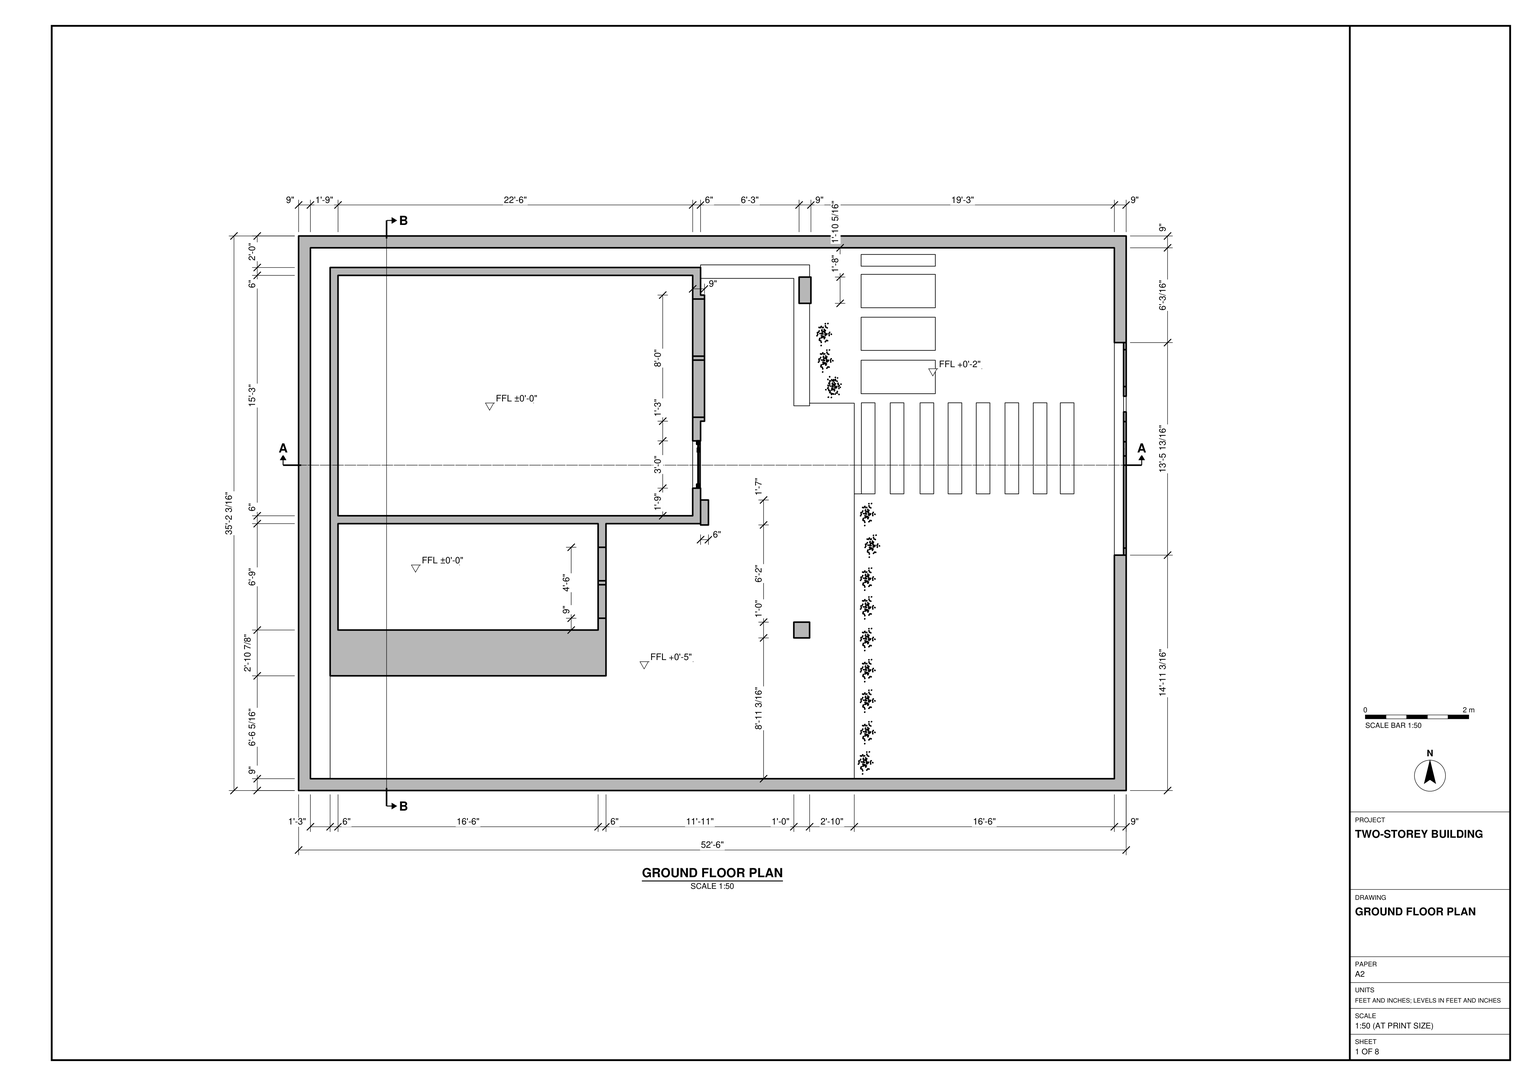
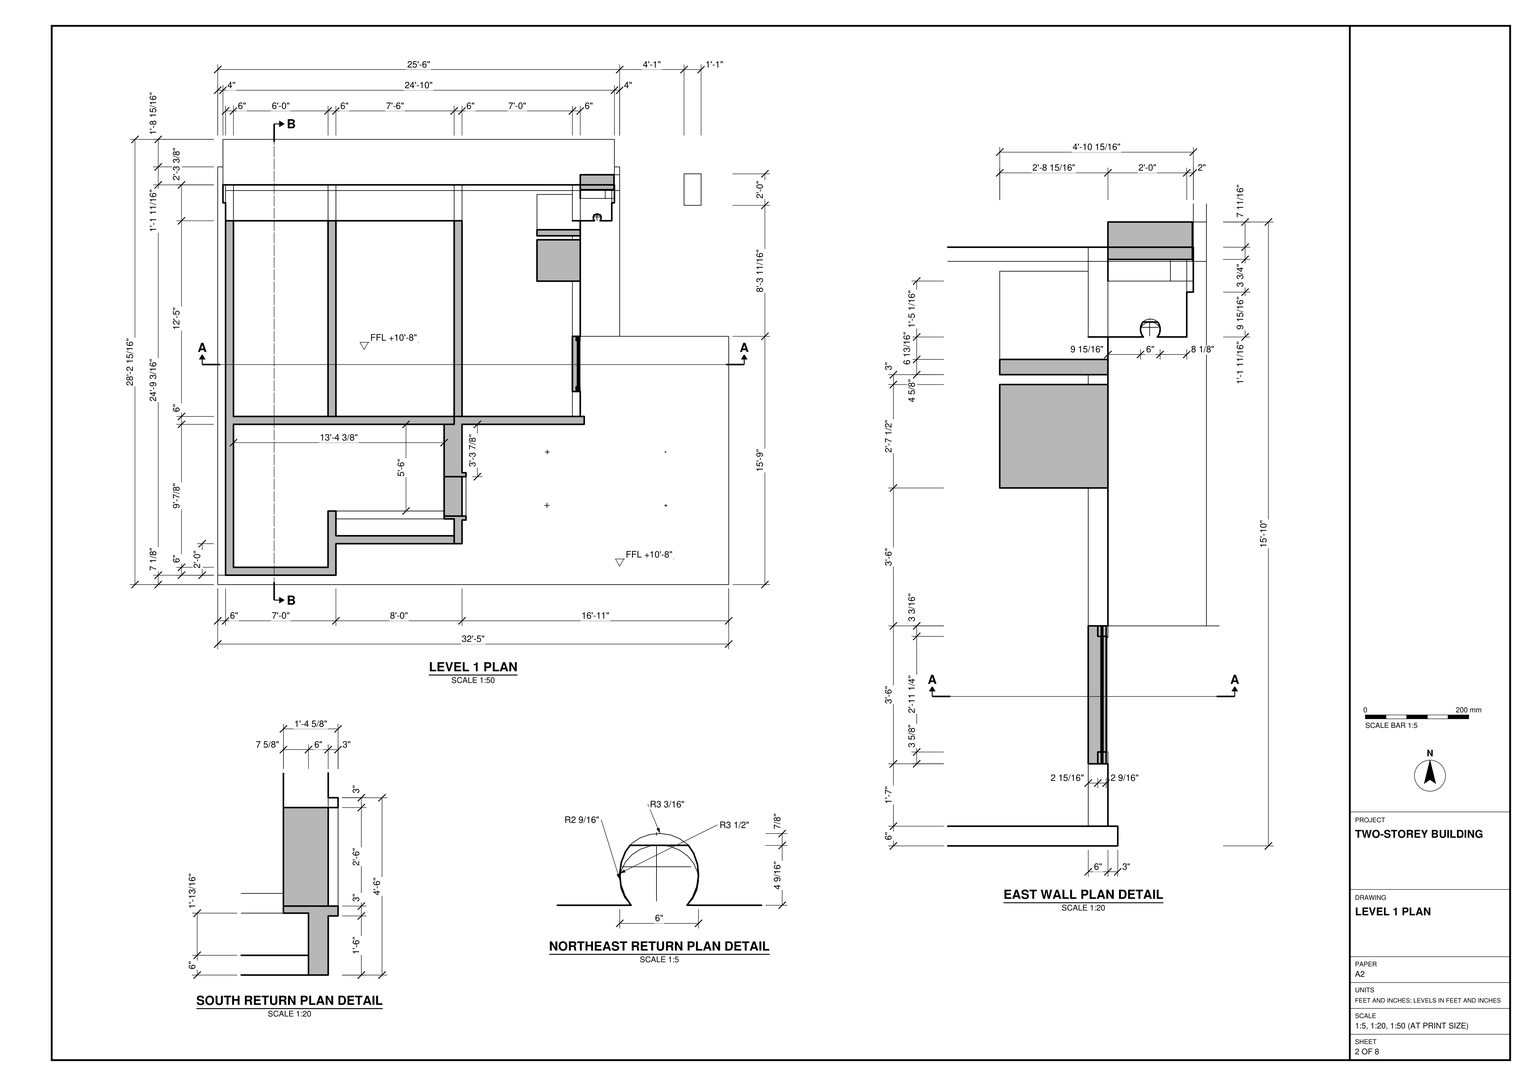
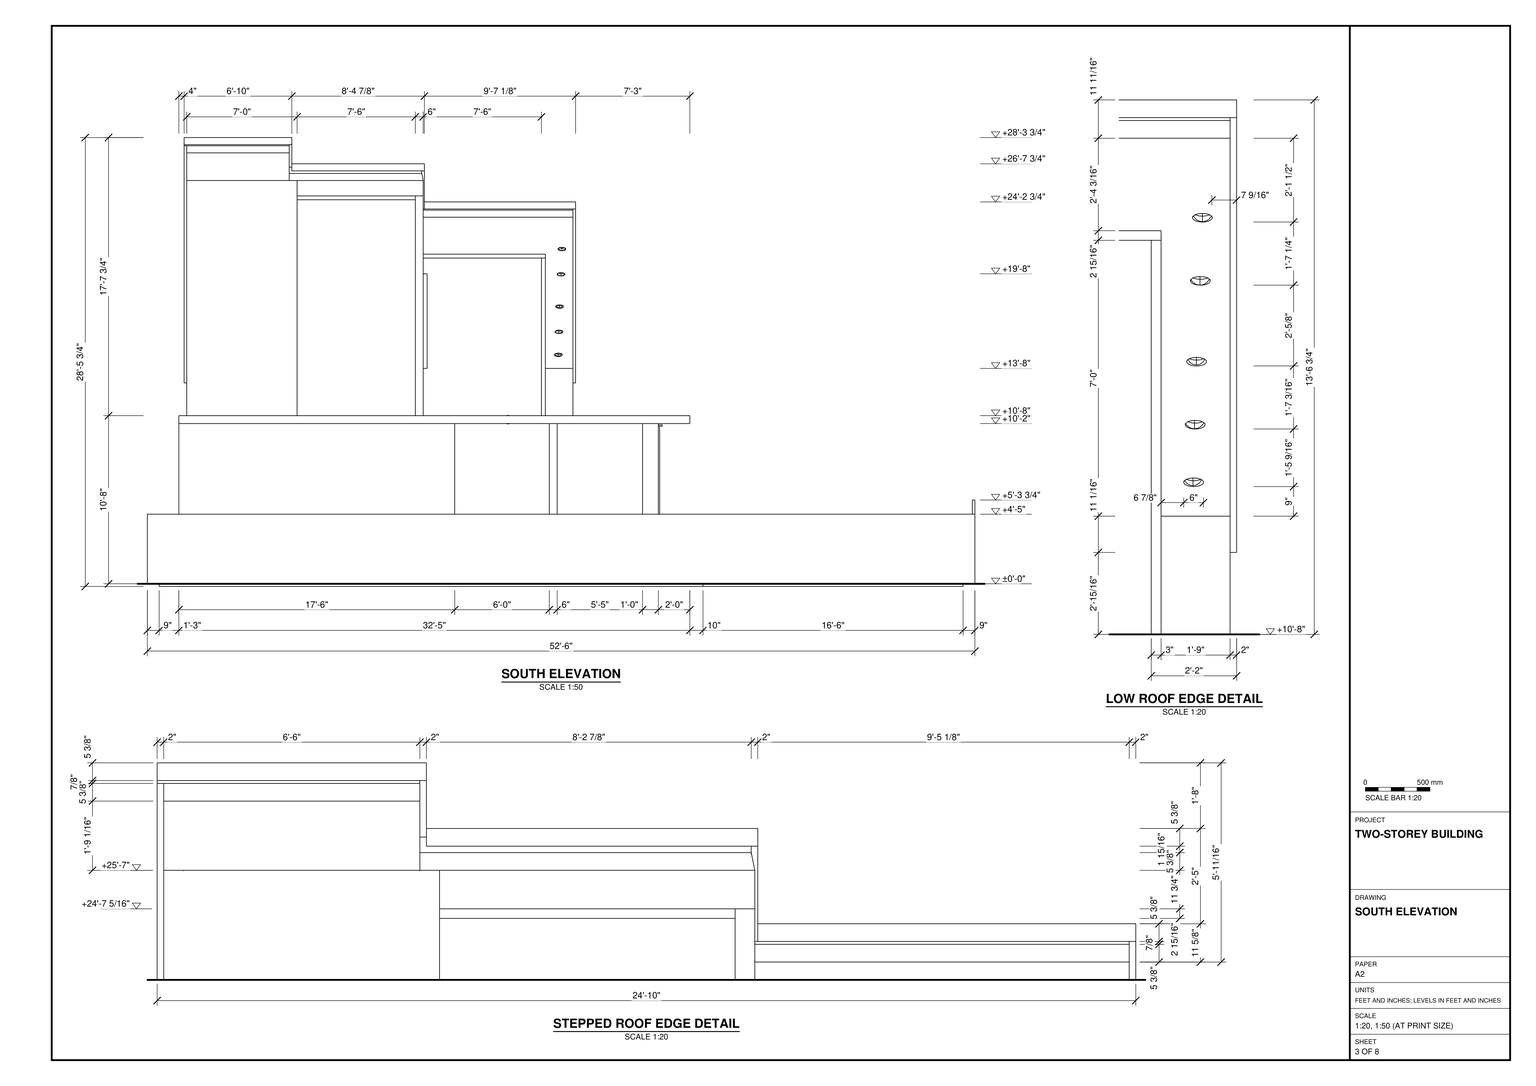
Build the two-storey building and its enclosed site in SketchUp using task_files/diagram_01.pdf. Work in feet and inches. The overall model extents, including the site walls, are 52'-6" east to west, 35'-2 3/16" north to south and 28'-5 3/4" high. Set the ground floor at ±0'-0" and the upper floor at +10'-8".

Place the building toward the west side of the site. Lay out the larger ground-floor room with the narrower room adjoining it to the south. Follow the plans for wall thicknesses, door and window openings, and changes in the exterior floor level. Model the upper-floor slab, including its projection beyond the enclosed rooms and the supports beneath it. Use the upper plan and its enlarged details for the partitions and wall returns. Shape the roof in three steps, using the south elevation for their relative heights and the edge detail for the projecting bands. Include the east boundary gate, the two runs of paving leading into the yard and the adjacent planted strip.

Keep walls, slabs and roofs in separate groups or components, and do the same for each furniture or joinery piece shown. Use components for repeated parts. Plants, lights and other loose or decorative items may be any suitable library components. Save one SketchUp model as output_files/two_storey_building_with_stepped_roofs_and_a_gated_yard.skp.

# SketchUp Ruby script. Lengths in inches.
U = 1.inch
M = Sketchup.active_model
def pt(a) = Geom::Point3d.new(a.map { |v| v * U })
def face(e, loops, mat)
  f = e.add_face(loops[0].map { |a| pt(a) })
  loops[1..].each { |l| e.add_face(l.map { |a| pt(a) }).erase! }
  f.material = f.back_material = mat if mat
  f
end
# faces: each face lists its corners as indices into pts; further lists are holes
def faces(e, pts, list, mat = nil) = list.each { |f| face(e, (f[0].is_a?(Array) ? f : [f]).map { |l| l.map { |i| pts[i] } }, mat) }
# xy, xz, yz: faces in a plane at the given z, y or x. An outline is a flat list of corners, or four numbers for a rectangle; further outlines are holes
def ring(l) = l.size == 4 ? [[l[0], l[1]], [l[2], l[1]], [l[2], l[3]], [l[0], l[3]]] : l.each_slice(2).to_a
def flat(e, list, mat, &to3) = list.each { |f| face(e, (f[0].is_a?(Array) ? f : [f]).map { |l| ring(l).map { |u, v| to3.(u, v) } }, mat) }
def xy(e, z, list, mat = nil) = flat(e, list, mat) { |x, y| [x, y, z] }
def xz(e, y, list, mat = nil) = flat(e, list, mat) { |x, z| [x, y, z] }
def yz(e, x, list, mat = nil) = flat(e, list, mat) { |y, z| [x, y, z] }
def lines(e, pts, list) = list.each { |a, b| e.add_line(pt(pts[a]), pt(pts[b])) }
# prism: a flat outline (further loops are holes) pulled along v
def prism(e, loops, v, mat = nil)
  f = face(e, loops, mat); d = Geom::Vector3d.new(v.map { |x| x * U })
  f.pushpull(f.normal.samedirection?(d) ? d.length : -d.length)
end
def box(e, o, s, mat = nil) = prism(e, [[o, [o[0] + s[0], o[1], o[2]], [o[0] + s[0], o[1] + s[1], o[2]], [o[0], o[1] + s[1], o[2]]]], [0, 0, s[2]], mat)
def at(x, y, z, deg = 0) = Geom::Transformation.translation(pt([x, y, z])) * Geom::Transformation.rotation(ORIGIN, Z_AXIS, deg.degrees)
def axes(o, x, y, z) = Geom::Transformation.new([*x, 0, *y, 0, *z, 0, *pt(o).to_a, 1])
def part(name) = M.definitions.add(name)
# library, detail: a bought-in or finely detailed component or shape, given as its bounding box
def library(name, o, s) = part(name).tap { |d| box(d.entities, o, s) }
def detail(e, o, s) = box(e.add_group.entities, o, s)
def put(e, d, t, mat = nil) = e.add_instance(d, t).tap { |i| i.material = mat if mat }
def group(e, t, mat = nil) = e.add_group.tap { |g| g.transformation = t; g.material = mat if mat }.entities
root = M.entities
M.materials.add("Asphalt_02_1K").color = [86, 76, 68]
M.materials.add("Concrete_04_1K").color = [254, 255, 241]
M.materials.add("D03_Lemon_Mist").color = [255, 216, 101]
M.materials.add("Glass_Basic_01").color = [253, 255, 84]
M.materials.add("LightPink_Translucent").color = [144, 107, 117]
M.materials.add("Marble_01_1K").color = [227, 230, 224]
M.materials.add("Marble_07_1K").color = [36, 34, 36]
M.materials.add("Plywood_01_1K").color = [130, 82, 50]
M.materials.add("Plywood_01_1K1").color = [125, 97, 41]
M.materials.add("Roofing_01_1K").color = [248, 255, 241]
M.materials.add("Roofing_01_1K1").color = [234, 220, 203]
M.materials.add("Roofing_02_1K").color = [97, 118, 74]
M.materials.add("ThomThom - Buttons1").color = [48, 49, 53]
M.materials.add("[Color_000]").color = [255, 255, 255]
c1 = library("porta+4",[0.2,-5.42,1.33],[46.55,4.72,83.21])
c2 = part("blade")
p = [[2.15,0.21,22],[0,0.17,0],[0.09,0.45,0],[2.18,0.31,22],[2.29,0.31,22],[0.38,0.45,0],
  [2.48,0.24,33],[2.49,0.24,33],[2.48,0.22,33]]
faces(c2.entities,p,[[0,1,2,3],[4,5,2,3],[6,3,4,7],[8,0,3,6]])
c3 = part("seeds")
p = [[0.3,-0.1,1.38],[-0.01,-0.03,1.59],[-0.01,-0.03,0.03],[0.14,-0.07,-0.07],[0.29,-0.03,3],[0.15,0.01,3.11]]
faces(c3.entities,p,[[0,1,2,3],[1,0,4,5]],"LightPink_Translucent")
c4 = part("blade with seeds")
put(c4.entities,c2,at(0,0,0))
put(c4.entities,c3,axes([2.4,0.25,30.99],[1.5799,-0.05474,1.17369],[-0.12525,1.92788,0.29478],[-0.07173,-0.02425,1.56792]))
c5 = part("Regal mist grass")
put(c5.entities,c4,axes([-3.26,-3.84,1.05],[0.05632,0.08194,0.78597],[-0.27153,0.73654,-0.07427],[-0.27499,0.00533,0.13909]))
put(c5.entities,c4,axes([-3.73,-1.59,0.19],[0.48504,-0.05875,0.50893],[-0.30767,0.51765,0.37393],[-0.23969,-0.07765,0.1121]))
put(c5.entities,c4,axes([-2.85,-2.28,0.11],[0.14833,0.22859,0.63362],[-0.3418,0.62134,-0.13627],[-0.35096,-0.14851,0.27091]))
put(c5.entities,c4,axes([3.2,1.81,0.97],[0.43228,0.51405,-0.15691],[-0.49359,0.48662,0.20258],[0.25079,0.07404,0.38762]))
put(c5.entities,c4,axes([2.7,2.1,0.19],[-0.42777,-0.23608,0.50893],[0.55235,-0.23987,0.37393],[0.14898,0.20319,0.1121]))
put(c5.entities,c4,axes([2.71,1.87,1.19],[0.04068,-0.83498,-0.05388],[0.77022,0.02282,-0.29906],[0.29664,0.058,0.45442]))
put(c5.entities,c4,axes([-3.45,-1.04,0.97],[-0.63139,-0.22904,-0.15691],[0.18416,-0.66822,0.20258],[-0.25421,0.06127,0.38762]))
put(c5.entities,c4,axes([-0.36,0.56,0.04],[0.20136,-0.97289,-0.10381],[0.95476,0.16959,0.22717],[-0.16683,-0.13435,0.69317]))
put(c5.entities,c4,axes([-2.43,-0.5,0.06],[0,0.82104,0.22],[-0.85,0,0],[0,-0.187,0.69788]))
put(c5.entities,c4,axes([1.82,-1.29,-0.13],[0.7903,0.13461,-0.27628],[-0.16677,0.83032,-0.07251],[0.23585,0.10061,0.60984]))
put(c5.entities,c4,axes([2.42,-3.36,0.01],[0.475,-0.82272,0],[0.79469,0.45881,-0.22867],[0.181,0.1045,0.72539]))
put(c5.entities,c4,axes([-2,3.05,0.45],[0.01669,-0.42385,0.68389],[0.75077,0.22388,0.09451],[-0.06505,0.45172,0.32293]))
put(c5.entities,c4,axes([-0.36,3.06,1.2],[-0.74862,-0.21464,0.23609],[0.25599,-0.70567,0.19467],[0.04499,0.27751,0.48853]))
put(c5.entities,c4,axes([-0.35,2.54,1.2],[0.22904,-0.63139,0.15691],[0.66822,0.18416,-0.20258],[0.06127,0.25421,0.38762]))
put(c5.entities,c4,axes([0.87,-4.07,1.06],[0.74862,0.21464,0.21269],[-0.25599,0.70567,0.17538],[-0.04499,-0.27751,0.44012]))
put(c5.entities,c4,axes([0.86,-3.55,1.2],[-0.22904,0.63139,0.15691],[-0.66822,-0.18416,-0.20258],[-0.06127,-0.25421,0.38762]))
put(c5.entities,c4,axes([-2.31,3.6875,0.11],[0.23975,-0.12952,0.63362],[0.59193,0.39053,-0.13627],[-0.17618,0.33792,0.27091]))
put(c5.entities,c4,axes([-0.89,-5.97,1.05],[-0.01417,0.09841,0.78597],[-0.69904,0.35716,-0.07427],[-0.20571,-0.18257,0.13909]))
put(c5.entities,c4,axes([2.82,2.98,-0.38],[0.05535,-0.11853,0.78135],[0.69686,-0.3491,-0.11937],[0.21127,0.18068,0.13309]))
put(c5.entities,c4,axes([0.6,3.36,1.05],[0.00225,-0.0994,0.78597],[0.65107,-0.43855,-0.07427],[0.22615,0.15653,0.13909]))
put(c5.entities,c4,axes([3.04,1.81,1.06],[-0.56019,0.541,0.21269],[-0.48313,-0.57453,0.17538],[0.26282,0.09979,0.44012]))
put(c5.entities,c4,axes([2.59,1.54,1.2],[-0.43228,-0.51405,0.15691],[0.49359,-0.48662,-0.20258],[0.25079,0.07404,0.38762]))
put(c5.entities,c4,axes([2.85,-2.86,-0.15],[0.71104,0.41052,-0.22],[-0.425,0.73612,0],[0.16194,0.0935,0.69788]))
put(c5.entities,c4,axes([-3.85,-0.6,1.05],[-0.12406,0.1066,0.77516],[0.01055,0.77884,-0.12259],[-0.28438,0.10128,0.06217]))
put(c5.entities,c4,axes([1.3,0.61,0.12],[0.56129,0.4933,0.06416],[-0.46819,0.55654,-0.18321],[-0.13032,0.07524,0.56159]))
put(c5.entities,c4,axes([1.125,0.43,0.14],[0.08853,0.93685,-0.12892],[-0.92207,0.05665,-0.22156],[-0.16237,0.12479,0.70765]))
put(c5.entities,c4,axes([-0.48,-0.93,-0.06],[0.36861,-0.73982,-0.19823],[0.76592,0.35605,0.0954],[0,-0.17054,0.63647]))
put(c5.entities,c4,axes([-3.05,-1.34,1.19],[0.38226,0.74345,-0.05388],[-0.67844,0.36535,-0.29906],[-0.2859,0.09809,0.45442]))
put(c5.entities,c4,axes([-0.85,-4.05,1.06],[0.3453,-0.52156,0.02849],[0.49172,0.30366,0.2243],[-0.15897,-0.16722,0.34202]))
put(c5.entities,c4,axes([-0.91,-3.46,1.17],[-0.64782,-0.39685,-0.31479],[0.4604,-0.69542,0.03799],[-0.23471,-0.23695,0.44531]))
put(c5.entities,c4,axes([5.64,-0.84,1.05],[0.10543,-0.12506,0.77516],[-0.13494,-0.76713,-0.12259],[0.26452,-0.14545,0.06217]))
put(c5.entities,c4,axes([0.86,-0.73,-0.0625],[0,-0.95,0],[0.95,0,0],[0,0,0.79515]))
put(c5.entities,c4,axes([1.65,0.49,0.68],[-0.2822,-0.14146,0.75935],[0.58401,-0.59344,0.0614],[0.36399,0.26771,0.32462]))
put(c5.entities,c4,axes([3.38,1.37,1.05],[0.16298,-0.01389,0.77516],[0.44703,-0.63786,-0.12259],[0.28989,0.0842,0.06217]))
put(c5.entities,c4,axes([3.82,0.11,1.06],[-0.21464,0.74862,0.21269],[-0.70567,-0.25599,0.17538],[0.27751,-0.04499,0.44012]))
put(c5.entities,c4,axes([3.3,0.1,1.2],[-0.63139,-0.22904,0.15691],[0.18416,-0.66822,-0.20258],[0.25421,-0.06127,0.38762]))
put(c5.entities,c4,axes([0.07,2.77,1.03],[0.74683,0.20582,-0.22641],[-0.25599,0.70567,-0.17538],[0.06848,0.28411,0.43322]))
put(c5.entities,c4,axes([-0.56,3.11,1.06],[-0.55982,0.27904,0.02849],[-0.27401,-0.50883,0.2243],[0.05406,0.2243,0.34202]))
put(c5.entities,c4,axes([-0.21,2.64,1.17],[0.36261,0.66759,-0.31479],[-0.74642,0.37205,0.03799],[0.08479,0.32256,0.44531]))
put(c5.entities,c4,axes([0.99,-1.65,0.12],[0.14656,-0.73274,0.06416],[0.71607,0.12719,-0.18321],[0.13032,0.07524,0.56159]))
put(c5.entities,c4,axes([1.74,-2.51,0.06],[-0.81639,0.21792,0.07817],[-0.20159,-0.81098,0.15546],[0.07281,0.11816,0.71074]))
put(c5.entities,c4,axes([1.48,-0.78,0.16],[0.36861,-0.73982,0.19823],[0.76592,0.35605,-0.0954],[0,0.17054,0.63647]))
put(c5.entities,c4,axes([0.64,1.03,0.43],[0.65653,0.33108,0.67022],[-0.64318,0.71325,0.26504],[-0.28809,-0.42273,0.56186]))
put(c5.entities,c4,axes([-3.14,0.74,1.06],[-0.18842,-0.75564,0.21269],[0.73912,-0.13114,0.17538],[-0.21784,0.17772,0.44012]))
put(c5.entities,c4,axes([-3.22,0.89,0.97],[-0.66132,0.11734,-0.15691],[-0.17463,-0.67077,0.20258],[-0.18951,0.18017,0.38762]))
put(c5.entities,c4,axes([-2.23,-2.48,1.17],[-0.75946,-0.01977,-0.31479],[0.05101,-0.83245,0.03799],[-0.32174,-0.08785,0.44531]))
put(c5.entities,c4,axes([-2.76,-3.02,1.22],[0.62742,-0.60592,0.23822],[0.54111,0.64347,0.19642],[-0.29436,-0.11177,0.49293]))
put(c5.entities,c4,axes([-2.08,-2.56,1.2],[0.43228,0.51405,0.15691],[-0.49359,0.48662,-0.20258],[-0.25079,-0.07404,0.38762]))
put(c5.entities,c4,axes([1.55,-0.55,0.14],[0.8556,0.39175,-0.12892],[-0.41198,0.82685,-0.22156],[0.02689,0.20301,0.70765]))
put(c5.entities,c4,axes([1.48,-0.16,-0.06],[0.53033,0.53033,0],[-0.53033,0.53033,0],[0,0,0.75]))
put(c5.entities,c4,axes([2.63,-2.96,1.19],[-0.83498,-0.04068,-0.05388],[0.02282,-0.77022,-0.29906],[0.058,-0.29664,0.45442]))
put(c5.entities,c4,axes([2.0625,-3.25,1.03],[-0.54387,-0.55166,-0.22641],[0.57453,-0.48313,-0.17538],[0.08275,-0.28029,0.43322]))
put(c5.entities,c4,axes([3.97,0.02,0.97],[0.63139,0.22904,-0.15691],[-0.18416,0.66822,0.20258],[0.25421,-0.06127,0.38762]))
put(c5.entities,c4,axes([4.49,1.89,0.7],[-0.14541,-0.69018,-0.01547],[0.68728,-0.15867,-0.07015],[0.14352,0.04375,0.23137]))
put(c5.entities,c4,axes([3.57,0.32,1.19],[-0.38226,-0.74345,-0.05388],[0.67844,-0.36535,-0.29906],[0.2859,-0.09809,0.45442]))
put(c5.entities,c4,axes([-1.14,-3.99,0.97],[-0.11734,-0.66132,-0.15691],[0.67077,-0.17463,0.20258],[-0.18017,-0.18951,0.38762]))
put(c5.entities,c4,axes([-0.04,-4.56,-0.1],[-0.52501,0.47102,-0.01725],[-0.48105,-0.51587,-0.0782],[-0.03387,-0.14617,0.25794]))
put(c5.entities,c4,axes([-0.69,-4.1,1.37],[-0.50704,0.78711,-0.06035],[-0.7343,-0.45346,-0.33495],[-0.25525,-0.22238,0.50895]))
put(c5.entities,c4,axes([-1.22,-3.44,1.03],[-0.74969,0.19517,-0.22641],[-0.13114,-0.73912,-0.17538],[-0.20136,-0.21181,0.43322]))
put(c5.entities,c4,axes([3.39,-4.18,1.05],[-0.00733,-0.1634,0.77516],[-0.61941,-0.47227,-0.12259],[0.09577,-0.28628,0.06217]))
put(c5.entities,c4,axes([-2.27,-0.88,-0.01],[-0.70668,0.69027,0.13628],[-0.70711,-0.68301,-0.16169],[-0.02468,-0.19603,0.73059]))
put(c5.entities,c4,axes([-0.42,0.16,-0.06],[-0.4564,-0.68913,-0.19823],[0.69131,-0.48528,0.0954],[-0.14769,-0.08527,0.63647]))
put(c5.entities,c4,axes([-1.79,1.83,1.2],[0.51405,-0.43228,0.15691],[0.48662,0.49359,-0.20258],[-0.07404,0.25079,0.38762]))
put(c5.entities,c4,axes([-2.14,3.0625,0.21],[0.69018,-0.14539,0.02883],[0.15867,0.58575,-0.38241],[-0.04375,0.29652,0.34277]))
put(c5.entities,c4,axes([-0.57,2.8,1.19],[0.74345,-0.38226,-0.05388],[0.36535,0.67844,-0.29906],[0.09809,0.2859,0.45442]))
put(c5.entities,c4,axes([-2.68,0.49,1.2],[0.66132,-0.11734,0.15691],[0.17463,0.67077,-0.20258],[-0.18951,0.18017,0.38762]))
put(c5.entities,c4,axes([-2.06,2.27,1.06],[-0.541,-0.56019,0.21269],[0.57453,-0.48313,0.17538],[-0.09979,0.26282,0.44012]))
put(c5.entities,c4,axes([1.29,-3.38,0.68],[-0.14146,0.2822,0.75935],[-0.59344,-0.58401,0.0614],[0.26771,-0.36399,0.32462]))
put(c5.entities,c4,axes([3.8,-1.61,1.06],[0.52156,0.3453,0.02849],[-0.30366,0.49172,0.2243],[0.16722,-0.15897,0.34202]))
put(c5.entities,c4,axes([3.21,-1.68,1.17],[0.39685,-0.64782,-0.31479],[0.69542,0.4604,0.03799],[0.23695,-0.23471,0.44531]))
put(c5.entities,c4,axes([4.29,-0.11,-0.16],[-0.48932,0.09853,0.62734],[-0.07789,-0.78429,0.03591],[0.34272,-0.11871,0.35698]))
put(c5.entities,c4,axes([-0.57,-0.3125,0.14],[-0.8556,-0.39175,-0.12892],[0.41198,-0.82685,-0.22156],[-0.02689,-0.20301,0.70765]))
put(c5.entities,c4,axes([-3.375,-0.75,-0.38],[0.01927,0.12939,0.78135],[-0.38842,0.67573,-0.11937],[-0.2759,-0.03406,0.13309]))
put(c5.entities,c4,axes([-3.83,2.3125,1.05],[-0.01889,0.16248,0.77516],[0.53593,0.56522,-0.12259],[-0.1403,0.26729,0.06217]))
put(c5.entities,c4,axes([-5.23,0.19,1.05],[0.09696,0.02202,0.78597],[0.29994,0.72543,-0.07427],[-0.19848,0.1904,0.13909]))
put(c5.entities,c4,axes([-1.08,-3.5625,0.01],[-0.475,-0.82272,0],[0.79469,-0.45881,-0.22867],[0.181,-0.1045,0.72539]))
put(c5.entities,c4,axes([-0.27,-3.37,-0.14],[0.70879,0.20315,-0.13726],[-0.17846,0.71541,0.13726],[0.14289,-0.0825,0.61578]))
put(c5.entities,c4,axes([3.53,-0.32,1.03],[0.20582,-0.74683,-0.22641],[0.70567,0.25599,-0.17538],[0.28411,-0.06848,0.43322]))
put(c5.entities,c4,axes([2.25,-0.8,0.68],[-0.31513,0.0186,0.75935],[0.20905,-0.80594,0.0614],[0.44908,0.04985,0.32462]))
put(c5.entities,c4,axes([3.875,0.31,1.06],[0.27904,0.55982,0.02849],[-0.50883,0.27401,0.2243],[0.2243,-0.05406,0.34202]))
put(c5.entities,c4,axes([3.4,-0.04,1.17],[0.66759,-0.36261,-0.31479],[0.37205,0.74642,0.03799],[0.32256,-0.08479,0.44531]))
put(c5.entities,c4,axes([-2.2,-2.88,1.19],[-0.04068,0.83498,-0.05388],[-0.77022,-0.02282,-0.29906],[-0.29664,-0.058,0.45442]))
put(c5.entities,c4,axes([-2.49,-2.3125,1.03],[-0.55166,0.54387,-0.22641],[-0.48313,-0.57453,-0.17538],[-0.28029,-0.08275,0.43322]))
put(c5.entities,c4,axes([0.49,1.3125,0.68],[-0.17367,-0.26361,0.75935],[0.80249,-0.22193,0.0614],[0.18137,0.41384,0.32462]))
put(c5.entities,c4,axes([-2.47,-3.02,1.06],[0.03826,-0.62433,0.02849],[0.57767,0.01712,0.2243],[-0.22128,-0.06533,0.34202]))
put(c5.entities,c4,axes([0.09,-5.13,-0.38],[-0.12743,0.02958,0.78135],[-0.70471,-0.33298,-0.11937],[0.01182,-0.27774,0.13309]))
put(c5.entities,c4,axes([1.8,-0.61,0.12],[0.70785,-0.23944,0.06416],[0.24789,0.68373,-0.18321],[0,0.15048,0.56159]))
put(c5.entities,c4,axes([2.92,-0.39,0.06],[-0.59691,-0.59805,0.07817],[0.60154,-0.58007,0.15546],[-0.06593,0.12214,0.71074]))
put(c5.entities,c4,axes([2.77,-3.23,1.06],[0.62433,0.03826,0.02849],[-0.01712,0.57767,0.2243],[0.06533,-0.22128,0.34202]))
put(c5.entities,c4,axes([-0.93,1.44,0.68],[-0.0186,-0.31513,0.75935],[0.80594,0.20905,0.0614],[-0.04985,0.44908,0.32462]))
put(c5.entities,c4,axes([2.23,-3,1.17],[0.01977,-0.75946,-0.31479],[0.83245,0.05101,0.03799],[0.08785,-0.32174,0.44531]))
put(c5.entities,c4,axes([-2.22,0.85,0.68],[0.14146,-0.2822,0.75935],[0.59344,0.58401,0.0614],[-0.26771,0.36399,0.32462]))
put(c5.entities,c4,axes([2.57,-3.29,1.06],[0.541,0.56019,0.21269],[-0.57453,0.48313,0.17538],[0.09979,-0.26282,0.44012]))
put(c5.entities,c4,axes([-0.83,0.43,-0.13],[-0.7903,-0.13461,-0.27628],[0.16677,-0.83032,-0.07251],[-0.23585,-0.10061,0.60984]))
put(c5.entities,c4,axes([1.17,1.85,0.11],[0.01341,-0.27217,0.63362],[0.64069,-0.30401,-0.13627],[0.19778,0.32575,0.27091]))
put(c5.entities,c4,axes([-3.05,-0.3125,0.68],[0.26361,-0.17367,0.75935],[0.22193,0.80249,0.0614],[-0.41384,0.18137,0.32462]))
put(c5.entities,c4,axes([0.55,4.79,1.46],[0.52501,-0.47102,-0.02875],[0.48105,0.51587,-0.13034],[0.03387,0.14617,0.4299]))
put(c5.entities,c4,axes([1.19,2.78,1.19],[0.45272,-0.70277,-0.05388],[0.65562,0.40488,-0.29906],[0.2279,0.19855,0.45442]))
put(c5.entities,c4,axes([3.41,0.38,-0.14],[-0.53033,0.51226,-0.13726],[-0.53033,-0.51226,0.13726],[0,0.165,0.61578]))
put(c5.entities,c4,axes([1.4,-1.03,-0.06],[0.4564,0.68913,-0.19823],[-0.69131,0.48528,0.0954],[0.14769,0.08527,0.63647]))
put(c5.entities,c4,axes([-4.42,2.5,0.19],[0.31662,-0.37211,0.50893],[0.12494,0.58908,0.37393],[-0.22881,0.10548,0.1121]))
put(c5.entities,c4,axes([2.01,-2.93,0.06],[-0.71104,-0.41052,0.22],[0.425,-0.73612,0],[0.16194,0.0935,0.69788]))
put(c5.entities,c4,axes([-2.08,0.23,0.68],[0.18976,-0.25227,0.75935],[0.47913,0.68094,0.0614],[-0.32863,0.3101,0.32462]))
put(c5.entities,c4,axes([-3.03,0.43,1.19],[0.70277,0.45272,-0.05388],[-0.40488,0.65562,-0.29906],[-0.19855,0.2279,0.45442]))
put(c5.entities,c4,axes([1.41,2.83,-0.15],[-0.71104,0.41052,-0.22],[-0.425,-0.73612,0],[-0.16194,0.0935,0.69788]))
put(c5.entities,c4,axes([0.92,0.8,0.05],[-0.74186,-0.66083,-0.11162],[0.62425,-0.74205,0.24427],[-0.19977,0.0773,0.74534]))
put(c5.entities,c4,axes([1.1,0,-0.02],[-0.70668,-0.70668,-0.02717],[0.70711,-0.70711,0],[-0.02468,-0.02468,0.77794]))
put(c5.entities,c4,axes([-2.8,-1.26,-0.15],[0,-0.82104,-0.22],[0.85,0,0],[0,-0.187,0.69788]))
put(c5.entities,c4,axes([1.34,-0.35,-0.02],[0,0.94953,-0.02498],[-0.95,0,0],[0,0.02984,0.79476]))
put(c5.entities,c4,axes([2.98,2.01,1.06],[-0.03826,0.62433,0.02849],[-0.57767,-0.01712,0.2243],[0.22128,0.06533,0.34202]))
put(c5.entities,c4,axes([-1.42,-3.85,0.68],[0.17367,0.26361,0.75935],[-0.80249,0.22193,0.0614],[-0.18137,-0.41384,0.32462]))
put(c5.entities,c4,axes([2.75,1.47,1.17],[0.75946,0.01977,-0.31479],[-0.05101,0.83245,0.03799],[0.32174,0.08785,0.44531]))
put(c5.entities,c4,axes([-0.4375,2.95,-0.38],[0.12296,-0.04468,0.78135],[0.7396,0.2459,-0.11937],[0.02163,0.27715,0.13309]))
put(c5.entities,c4,axes([1.25,2.43,1.2],[-0.11734,-0.66132,0.15691],[0.67077,-0.17463,-0.20258],[0.18017,0.18951,0.38762]))
put(c5.entities,c4,axes([1.46,2.61,-0.07],[-0.46908,-0.8256,-0.02278],[0.79469,-0.45881,0.22867],[-0.19583,0.0786,0.72503]))
put(c5.entities,c4,axes([1.48,2.1875,-0.01],[0.95113,0.26686,0.13628],[-0.23795,0.95388,-0.16169],[-0.15742,0.11938,0.73059]))
put(c5.entities,c4,axes([1.71,-1.37,0.94],[-0.65649,-0.4266,0.61271],[0.6932,-0.66419,0.26437],[0.21181,0.40027,0.59225]))
put(c5.entities,c4,axes([3.61,0.25,-0.07],[-0.94953,-0.00656,-0.02205],[0,-0.91763,0.22129],[-0.02984,0.20889,0.70164]))
put(c5.entities,c4,axes([-1.67,1.69,-0.14],[-0.17846,-0.71541,-0.13726],[0.70879,-0.20315,0.13726],[-0.14289,-0.0825,0.61578]))
put(c5.entities,c4,axes([-2.12,1.95,1.35],[0.83498,0.04068,-0.05981],[-0.02282,0.77022,-0.33196],[-0.058,0.29664,0.5044]))
put(c5.entities,c4,axes([-3.28,0.6,1.06],[-0.52156,-0.3453,0.02849],[0.30366,-0.49172,0.2243],[-0.16722,0.15897,0.34202]))
put(c5.entities,c4,axes([-2.68,0.97,1.03],[0.19517,0.74969,-0.22641],[-0.73912,0.13114,-0.17538],[-0.21181,0.20136,0.43322]))
put(c5.entities,c4,axes([-3.02,-0.7,1.03],[-0.20582,0.74683,-0.22641],[-0.70567,-0.25599,-0.17538],[-0.28411,0.06848,0.43322]))
put(c5.entities,c4,axes([-0.75,4.32,1.05],[0.0963,0.13221,0.77516],[0.77718,0.05194,-0.12259],[0.07815,0.29158,0.06217]))
put(c5.entities,c4,axes([-0.25,0.09,0.01],[0.96024,0.17298,0.20273],[-0.19542,0.97698,0.07956],[-0.14033,-0.09434,0.70387]))
put(c5.entities,c4,axes([3.41,-0.36,0.06],[0,-0.82104,0.22],[0.85,0,0],[0,0.187,0.69788]))
put(c5.entities,c4,axes([1.46,0.0625,-0.06],[-0.36861,0.73982,-0.19823],[-0.76592,-0.35605,0.0954],[0,0.17054,0.63647]))
put(c5.entities,c4,axes([-2.58,-3.03,0.68],[0.2822,0.14146,0.75935],[-0.58401,0.59344,0.0614],[-0.36399,-0.26771,0.32462]))
put(c5.entities,c4,axes([5.27,-1.64,1.05],[-0.09923,-0.00624,0.78597],[-0.41207,-0.66814,-0.07427],[0.16548,-0.21969,0.13909]))
put(c5.entities,c4,axes([-1.55,2.24,1.18],[0.54387,0.55166,-0.25132],[-0.57453,0.48313,-0.19467],[-0.08275,0.28029,0.48087]))
put(c5.entities,c4,axes([-2.06,2.44,0.97],[-0.51405,0.43228,-0.15691],[-0.48662,-0.49359,0.20258],[-0.07404,0.25079,0.38762]))
put(c5.entities,c4,axes([-1.87,2,-0.15],[-0.71104,-0.41052,-0.22],[0.425,-0.73612,0],[-0.16194,-0.0935,0.69788]))
put(c5.entities,c4,axes([5.09,2.53,1.05],[-0.0687,-0.07188,0.78597],[0.15027,-0.77048,-0.07427],[0.2706,-0.04923,0.13909]))
put(c5.entities,c4,axes([0.88,1.48,-0.02],[0.33031,0.94323,-0.02664],[-0.9438,0.33051,0],[0.01153,0.03294,0.76288]))
put(c5.entities,c4,axes([1.39,1.36,-0.07],[0.79762,-0.27858,-0.08506],[0.28027,0.80246,0.00004],[0.08804,-0.03079,0.77052]))
put(c5.entities,c4,axes([5.31,0.16,0.19],[-0.46941,0.13554,0.50893],[0.22095,-0.56018,0.37393],[0.24902,0.03833,0.1121]))
put(c5.entities,c4,axes([0.46,1.46,-0.0625],[-0.24789,-0.70785,0],[0.70785,-0.24789,0],[0,0,0.684]))
put(c5.entities,c4,axes([1.71,-4.23,0.11],[-0.21596,0.16619,0.63362],[-0.64676,-0.29087,-0.13627],[0.11989,-0.36174,0.27091]))
put(c5.entities,c4,axes([1.16,1.79,-0.0625],[0.76592,0.36861,0],[-0.36861,0.76592,0],[0,0,0.7752]))
put(c5.entities,c4,axes([3.79,-2.27,0.11],[-0.27141,-0.02432,0.63362],[-0.27805,-0.65237,-0.13627],[0.33343,-0.18455,0.27091]))
put(c5.entities,c4,axes([4.82,-0.62,-0.38],[-0.03971,-0.12465,0.78135],[0.27539,-0.72914,-0.11937],[0.27779,-0.01049,0.13309]))
put(c5.entities,c4,axes([1.09,-3.82,1.19],[-0.74345,0.38226,-0.05388],[-0.36535,-0.67844,-0.29906],[-0.09809,-0.2859,0.45442]))
put(c5.entities,c4,axes([0.45,-3.79,1.03],[-0.74683,-0.20582,-0.22641],[0.25599,-0.70567,-0.17538],[-0.06848,-0.28411,0.43322]))
put(c5.entities,c4,axes([1.07,-4.125,1.06],[0.55982,-0.27904,0.02849],[0.27401,0.50883,0.2243],[-0.05406,-0.2243,0.34202]))
put(c5.entities,c4,axes([0.72,-3.65,1.17],[-0.36261,-0.66759,-0.31479],[0.74642,-0.37205,0.03799],[-0.08479,-0.32256,0.44531]))
put(c5.entities,c4,axes([0.55,0.66,-0.06],[-0.82501,0.05068,-0.19823],[-0.07461,-0.84133,0.0954],[-0.14769,0.08527,0.63647]))
put(c5.entities,c4,axes([-1.4375,2.49,0.01],[-0.475,0.82272,0],[-0.79469,-0.45881,-0.22867],[-0.181,-0.1045,0.72539]))
put(c5.entities,c4,axes([2.06,2.7,0.01],[0.475,0.82272,0],[-0.79469,0.45881,-0.22867],[-0.181,0.1045,0.72539]))
put(c5.entities,c4,axes([1.25,2.5,-0.14],[-0.70879,-0.20315,-0.13726],[0.17846,-0.71541,0.13726],[-0.14289,0.0825,0.61578]))
put(c5.entities,c4,axes([-4.18,2.4,1.46],[0.67042,0.21916,-0.02875],[-0.20623,0.67454,-0.13034],[-0.10965,0.10242,0.4299]))
put(c5.entities,c4,axes([-1.87,-4.98,0.19],[0.39631,0.28576,0.50893],[-0.57716,0.17178,0.37393],[-0.12349,-0.21962,0.1121]))
put(c5.entities,c4,axes([-1.64,-4.54,0.11],[-0.04601,0.26859,0.63362],[-0.67257,0.22484,-0.13627],[-0.15721,-0.34715,0.27091]))
put(c5.entities,c4,axes([-3.36,-1.32,1.06],[-0.27904,-0.55982,0.02849],[0.50883,-0.27401,0.2243],[-0.2243,0.05406,0.34202]))
put(c5.entities,c4,axes([-0.3,-1.11,0.16],[-0.82501,0.05068,0.19823],[-0.07461,-0.84133,-0.0954],[0.14769,-0.08527,0.63647]))
put(c5.entities,c4,axes([0.41,-1.33,0.01],[-0.62993,0.7451,0.20273],[-0.74838,-0.65773,0.07956],[0.15186,-0.07436,0.70387]))
put(c5.entities,c4,axes([0.41,-2.01,-0.13],[0.51173,-0.61712,-0.27628],[0.63569,0.55959,-0.07251],[0.20505,-0.15394,0.60984]))
put(c5.entities,c4,axes([-1.53,-1.15,0.44],[0.21595,-0.11877,0.78455],[0.07447,0.82927,0.0614],[-0.46776,0.11004,0.2804]))
put(c5.entities,c4,axes([1.65,-0.55,0.22],[-0.02075,-0.77304,0.62596],[0.93928,0.20038,0.26504],[-0.22215,0.423,0.59086]))
put(c5.entities,c4,axes([-0.15,-1.29,0.14],[-0.08853,-0.93685,-0.12892],[0.92207,-0.05665,-0.22156],[0.16237,-0.12479,0.70765]))
put(c5.entities,c4,axes([-0.43,-3.69,-0.15],[0.71104,-0.41052,-0.22],[0.425,0.73612,0],[0.16194,-0.0935,0.69788]))
put(c5.entities,c4,axes([5.18,-0.8,-0.04],[-0.47102,-0.52501,-0.02875],[0.51587,-0.48105,-0.13034],[0.14617,-0.03387,0.4299]))
put(c5.entities,c4,axes([3.54,-1.44,1.19],[-0.70277,-0.45272,-0.05388],[0.40488,-0.65562,-0.29906],[0.19855,-0.2279,0.45442]))
put(c5.entities,c4,axes([3.19,-1.98,1.03],[-0.19517,-0.74969,-0.22641],[0.73912,-0.13114,-0.17538],[0.21181,-0.20136,0.43322]))
put(c5.entities,c4,axes([4.43,1.06,0.11],[-0.18297,-0.20193,0.63362],[0.23807,-0.668,-0.13627],[0.37019,0.09049,0.27091]))
put(c5.entities,c4,axes([3.74,-1.9,0.97],[0.66132,-0.11734,-0.15691],[0.17463,0.67077,0.20258],[0.18951,-0.18017,0.38762]))
put(c5.entities,c4,axes([-3.89,3.98,1.05],[0.08619,-0.04957,0.78597],[0.71239,0.32972,-0.07427],[-0.01674,0.27453,0.13909]))
put(c5.entities,c4,axes([-1.73,4.12,0.19],[-0.01966,-0.48819,0.50893],[0.49131,0.3482,0.37393],[-0.09662,0.23269,0.1121]))
put(c5.entities,c4,axes([-3.18,-1.73,0.68],[0.31513,-0.0186,0.75935],[-0.20905,0.80594,0.0614],[-0.44908,-0.04985,0.32462]))
put(c5.entities,c4,axes([1.73,2.43,1.03],[0.74969,-0.19517,-0.22641],[0.13114,0.73912,-0.17538],[0.20136,0.21181,0.43322]))
put(c5.entities,c4,axes([1.36,3.03,1.06],[-0.3453,0.52156,0.02849],[-0.49172,-0.30366,0.2243],[0.15897,0.16722,0.34202]))
put(c5.entities,c4,axes([2.76,3.18,0.14],[-0.48719,-0.02575,0.46551],[0.32174,-0.54689,0.25702],[0.19246,0.1943,0.36515]))
put(c5.entities,c4,axes([-0.01,0.79,0.12],[-0.14656,0.73274,0.06416],[-0.71607,-0.12719,-0.18321],[-0.13032,-0.07524,0.56159]))
put(c5.entities,c4,axes([0.68,-1.46,0.16],[-0.4564,-0.68913,0.19823],[0.69131,-0.48528,-0.0954],[0.14769,0.08527,0.63647]))
put(c5.entities,c4,axes([1.23,-0.95,0.02],[-0.96024,-0.17298,0.21799],[0.19542,-0.97698,0.08554],[0.14033,0.09434,0.75685]))
put(c5.entities,c4,axes([-0.5,-0.09,0.16],[-0.36861,0.73982,0.19823],[-0.76592,-0.35605,-0.0954],[0,-0.17054,0.63647]))
put(c5.entities,c4,axes([4.1,-3.47,0.19],[-0.25305,0.41795,0.50893],[-0.21751,-0.56153,0.37393],[0.209,-0.14071,0.1121]))
put(c5.entities,c4,axes([1.9,0.29,-0.11],[0.27858,0.75173,-0.30667],[-0.80246,0.27073,-0.08049],[0.03079,0.25455,0.67692]))
put(c5.entities,c4,axes([3.99,-0.22,0.01],[0.95,0,0],[0,0.91763,-0.22867],[0,0.209,0.72539]))
put(c5.entities,c4,axes([-0.33,-0.81,0.01],[0.33031,0.91809,0.20273],[-0.9438,0.31925,0.07956],[0.01153,-0.1687,0.70387]))
put(c5.entities,c4,axes([2.65,-2.56,-0.14],[0.17846,0.71541,-0.13726],[-0.70879,0.20315,0.13726],[0.14289,0.0825,0.61578]))
put(c5.entities,c4,axes([-2.18,-4.12,-0.38],[-0.07359,0.10816,0.78135],[-0.74371,0.23319,-0.11937],[-0.17966,-0.21213,0.13309]))
put(c5.entities,c4,axes([1.89,2.13,0.06],[0.71104,-0.41052,0.22],[0.425,0.73612,0],[-0.16194,0.0935,0.69788]))
put(c5.entities,c4,axes([0.92,-1.41,0.14],[0.76707,-0.54509,-0.12892],[0.51009,0.77021,-0.22156],[0.18926,0.07822,0.70765]))
put(c5.entities,c4,axes([0.0625,0.55,0.14],[-0.76707,0.54509,-0.12892],[-0.51009,-0.77021,-0.22156],[-0.18926,-0.07822,0.70765]))
put(c5.entities,c4,axes([-3.31,-1.12,1.06],[0.21464,-0.74862,0.21269],[0.70567,0.25599,0.17538],[-0.27751,0.04499,0.44012]))
put(c5.entities,c4,axes([0.57,1.15,-0.13],[-0.51173,0.61712,-0.27628],[-0.63569,-0.55959,-0.07251],[-0.20505,0.15394,0.60984]))
put(c5.entities,c4,axes([-1.03,2.06,0.06],[0.71104,0.41052,0.22],[-0.425,0.73612,0],[-0.16194,-0.0935,0.69788]))
put(c5.entities,c4,axes([-3.87,1.05,0.11],[0.26403,0.0674,0.63362],[0.17017,0.68843,-0.13627],[-0.35864,0.12887,0.27091]))
put(c5.entities,c4,axes([-3.58,2.88,-0.38],[0.10191,0.08203,0.78135],[0.1728,0.76002,-0.11937],[-0.22586,0.16207,0.13309]))
put(c5.entities,c4,axes([-0.28,3.2,0.97],[-0.22904,0.63139,-0.15691],[-0.66822,-0.18416,0.20258],[0.06127,0.25421,0.38762]))
put(c5.entities,c4,axes([3.23,-4.77,1.05],[-0.07716,0.06271,0.78597],[-0.75594,-0.21158,-0.07427],[-0.02737,-0.27368,0.13909]))
put(c5.entities,c4,axes([0.91,-5.55,0.19],[0.09746,0.47877,0.50893],[-0.54066,-0.26517,0.37393],[0.05818,-0.24515,0.1121]))
put(c5.entities,c4,axes([-0.09,-5.6,1.05],[-0.1162,-0.11512,0.77516],[-0.77549,0.07298,-0.12259],[-0.12377,-0.27534,0.06217]))
put(c5.entities,c4,axes([3.21,-3.72,-0.38],[-0.11371,-0.06468,0.78135],[-0.29209,-0.72261,-0.11937],[0.19704,-0.1961,0.13309]))
put(c5.entities,c4,axes([0.29,1.78,-0.07],[-0.76592,-0.36861,0],[0.36861,-0.76592,0],[0,0,0.72094]))
put(c5.entities,c4,axes([-0.6875,-2.56,0.06],[-0.21947,0.81597,0.07817],[-0.80313,-0.23091,0.15546],[0.13874,-0.00397,0.71074]))
put(c5.entities,c4,axes([1.67,1.7,0.06],[0.21947,-0.81597,0.07817],[0.80313,0.23091,0.15546],[-0.13874,0.00397,0.71074]))
put(c5.entities,c4,axes([1.28,0.25,0.16],[0.82501,-0.05068,0.19823],[0.07461,0.84133,-0.0954],[-0.14769,0.08527,0.63647]))
put(c5.entities,c4,axes([1.5,-0.52,-0.0625],[0.85,0,0],[0,0.85,0],[0,0,0.7905]))
put(c5.entities,c4,axes([3.65,-1.76,1.06],[0.18842,0.75564,0.21269],[-0.73912,0.13114,0.17538],[0.21784,-0.17772,0.44012]))
put(c5.entities,c4,axes([3.2,-1.51,1.2],[-0.66132,0.11734,0.15691],[-0.17463,-0.67077,-0.20258],[0.18951,-0.18017,0.38762]))
put(c5.entities,c4,axes([2.57,-3.46,0.97],[0.51405,-0.43228,-0.15691],[0.48662,0.49359,0.20258],[0.07404,-0.25079,0.38762]))
put(c5.entities,c4,axes([-2.79,-1.11,1.2],[0.63139,0.22904,0.15691],[-0.18416,0.66822,-0.20258],[-0.25421,0.06127,0.38762]))
put(c5.entities,c4,axes([-0.96,-1.14,-0.11],[-0.31201,-0.84193,-0.30943],[0.89876,-0.30322,-0.08121],[-0.03449,-0.2851,0.68302]))
put(c5.entities,c4,axes([2.3,-2.84,1.2],[-0.51405,0.43228,0.15691],[-0.48662,-0.49359,-0.20258],[0.07404,-0.25079,0.38762]))
put(c5.entities,c4,axes([0.79,-4.22,0.97],[0.22904,-0.63139,-0.15691],[0.66822,0.18416,0.20258],[-0.06127,-0.25421,0.38762]))
put(c5.entities,c4,axes([-1.72,1.98,1.33],[-0.01977,0.75946,-0.34942],[-0.83245,-0.05101,0.04217],[-0.08785,0.32174,0.49429]))
put(c5.entities,c4,axes([-2.26,2.22,1.06],[-0.62433,-0.03826,0.02849],[0.01712,-0.57767,0.2243],[-0.06533,0.22128,0.34202]))
put(c5.entities,c4,axes([-1.04,-4.23,1.22],[0.84632,-0.21103,0.23822],[0.14688,0.82782,0.19642],[-0.19904,-0.24398,0.49293]))
put(c5.entities,c4,axes([-0.74,-3.45,1.2],[0.11734,0.66132,0.15691],[-0.67077,0.17463,-0.20258],[-0.18017,-0.18951,0.38762]))
put(c5.entities,c4,axes([-2.69,-2.82,0.97],[-0.43228,-0.51405,-0.15691],[0.49359,-0.48662,0.20258],[-0.25079,-0.07404,0.38762]))
put(c5.entities,c4,axes([-2.65,-3.7,-0.1],[-0.21916,0.67042,-0.01725],[-0.67454,-0.20623,-0.0782],[-0.10242,-0.10965,0.25794]))
put(c5.entities,c4,axes([3.78,0.4,-0.15],[0,0.82104,-0.22],[-0.85,0,0],[0,0.187,0.69788]))
put(c5.entities,c4,axes([-0.76,1.65,0.06],[0.81639,-0.21792,0.07817],[0.20159,0.81098,0.15546],[-0.07281,-0.11816,0.71074]))
put(c5.entities,c4,axes([-0.03,-0.56,0.04],[0.85602,0.39794,0.10663],[-0.41198,0.82685,0.22156],[0,-0.1906,0.71135]))
put(c5.entities,c4,axes([-3.01,-0.64,0.01],[-0.95,0,0],[0,-0.91763,-0.22867],[0,-0.209,0.72539]))
put(c5.entities,c4,axes([-2.43,-1.24,-0.14],[0.53033,-0.51226,-0.13726],[0.53033,0.51226,0.13726],[0,-0.165,0.61578]))
put(c5.entities,c4,axes([-2.64,-4.33,1.05],[-0.16347,-0.0058,0.77516],[-0.52042,0.57954,-0.12259],[-0.27768,-0.11842,0.06217]))
put(c5.entities,c4,axes([1.51,2.89,1.06],[-0.75564,0.18842,0.21269],[-0.13114,-0.73912,0.17538],[0.17772,0.21784,0.44012]))
put(c5.entities,c4,axes([-1.02,-1.9,-0.33],[-0.74781,0.32871,0.57127],[-0.23802,-0.94316,0.22197],[0.4592,0.01569,0.64975]))
c6 = library("Modern+Gate+1",[0,0,0],[118.11,1.97,78.74])
c7 = library("Group\#2",[0,-71.98,-117],[389,374.91,334.75])
xy(root,-4,[[9,9,621,413.18]],"Roofing_02_1K")
xy(root,-2,[[0,0,0,422.18,630,422.18,630,341.02,621,341.02,621,413.18,9,413.18,9,9,621,9,621,179.2,630,179.2,630,0],[621,179.2,630,341.02]])
xy(root,0,[[428.41,225.85,438.8125,295.18],[450.39,225.85,460.8,295.18],[473.09,225.85,483.5,295.18],[494.45,225.85,504.85,295.18],[515.86,225.85,526.26,295.18],
  [537.75,225.85,548.15,295.18],[559.25,225.85,569.66,295.18],[579.86,225.85,590.27,295.18],[428.21,302.1,484.72,327.6],[428.21,335.07,484.72,360.33],
  [428.21,367.55,484.72,392.98],[428.21,399.17,484.72,408.11]],"Concrete_04_1K")
xy(root,51,[[0,0,630,0,630,179.2,621,179.2,621,9,9,9,9,413.18,621,413.18,621,341.02,630,341.02,630,422.18,0,422.18]],"Marble_07_1K")
xz(root,0,[[0,-2,630,51]],"Marble_07_1K")
xz(root,9,[[9,-4,423,-2]])
xz(root,9,[[9,-2,621,51]],"Marble_07_1K")
xz(root,9,[[423,-4,621,-2]],"Roofing_01_1K1")
xz(root,179.2,[[621,-2,630,51]],"Marble_07_1K")
xz(root,341.02,[[621,-2,630,51]],"Marble_07_1K")
xz(root,413.18,[[9,-4,387,-2]])
xz(root,413.18,[[9,-2,621,51]],"Marble_07_1K")
xz(root,413.18,[[387,-4,621,-2]],"Roofing_02_1K")
xz(root,422.18,[[0,-2,630,51]],"Marble_07_1K")
yz(root,0,[[0,-2,422.18,51]],"Marble_07_1K")
yz(root,9,[[9,-4,413.18,-2]])
yz(root,9,[[9,-2,413.18,51]],"Marble_07_1K")
yz(root,621,[[341.02,-2,413.18,51]])
yz(root,621,[[9,-2,179.2,51]],"Marble_07_1K")
yz(root,621,[[9,-4,179.2,-2],[179.2,-4,225.85,-2]],"Roofing_01_1K1")
yz(root,621,[[225.85,-4,294.89,-2],[294.89,-4,341.02,-2],[341.02,-4,413.18,-2]],"Roofing_02_1K")
yz(root,630,[[0,-2,179.2,51],[341.02,-2,422.18,51]],"Marble_07_1K")
# 4 loose lines left out
p = [[305.66,263.57,36.875],[305.66,233.28,36.875],[305.71,233.28,31.86],[305.71,263.57,31.86],[305.33,263.57,66.67],[305.33,233.28,66.67],
  [305.4,233.28,59.8],[305.4,263.57,59.8],[299.65,266,157.55],[299.65,230.78,157.55],[299.73,230.78,150.125],[299.73,266,150.125],
  [299.37,266,182.76],[299.37,230.78,182.76],[299.48,230.78,172.83],[299.48,266,172.83]]
faces(root,p,[[0,1,2,3],[4,5,6,7],[8,9,10,11],[12,13,14,15]],"Glass_Basic_01")
put(root,c1,axes([307.84,266.46,4.63],[0,-0.77596,0],[1,0,0],[0,0,0.99642]))
put(root,c5,axes([430.75,21.66,0.02],[0.49529,0,0],[0,0.67207,0],[0,0,1.94092]))
put(root,c5,axes([432.38,44.71,0.02],[0.49529,0,0],[0,0.67207,0],[0,0,1.94092]))
put(root,c5,axes([432.38,68.71,0.02],[0.49529,0,0],[0,0.67207,0],[0,0,1.94092]))
put(root,c5,axes([432.38,91.92,0.02],[0.49529,0,0],[0,0.67207,0],[0,0,1.94092]))
put(root,c5,axes([432.38,115.6,0.02],[0.49529,0,0],[0,0.67207,0],[0,0,1.94092]))
put(root,c5,axes([432.38,139.71,0.02],[0.49529,0,0],[0,0.67207,0],[0,0,1.94092]))
put(root,c5,axes([432.38,161.57,0.02],[0.49529,0,0],[0,0.67207,0],[0,0,1.94092]))
put(root,c5,axes([435.83,186.66,0.02],[0.49529,0,0],[0,0.67207,0],[0,0,1.94092]))
put(root,c5,axes([432.38,210.76,0.02],[0.49529,0,0],[0,0.67207,0],[0,0,1.94092]))
put(root,c5,axes([406.9,307.55,5.02],[0.49529,0,0],[0,0.67207,0],[0,0,1.94092]))
put(root,c5,axes([400.35,327.65,0.02],[0.49529,0,0],[0,0.67207,0],[0,0,1.94092]))
put(root,c5,axes([399.19,347.8,0.02],[0.49529,0,0],[0,0.67207,0],[0,0,1.94092]))
put(root,c6,axes([630,179.2,-2],[0,1.37007,0],[-1,0,0],[0,0,0.81]))
put(root,c7,at(24,116.18,120),"Asphalt_02_1K")
g1 = group(root,at(15,107.18,0),"D03_Lemon_Mist")
xy(g1,-2,[[[9,-98.18,408,-98.18,408,187.71,372,187.71,372,263.71,375,263.71,375,283.71,372,283.71,372,291,9,291],[15,15,15,96,213,96,213,102,15,102,15,285,285,285,285,102,213,102,213,15]],[15,15,213,96],[15,102,285,285]])
xy(g1,3,[[9,-98.18,408,-98.18,408,187.71,363,187.71,363,283.71,291,283.71,291,114,297,114,297,95,291,95,291,96,219,96,219,-19.85,9,-19.85]],"Marble_01_1K")
xy(g1,6,[[285,123,291,159]],"Plywood_01_1K")
xy(g1,27,[[291,174,294,270]],"Plywood_01_1K")
xy(g1,30,[[213,24,219,49.5]])
xy(g1,30,[[213,52.5,219,78],[285,177,294,220.5],[285,223.5,294,267]],"Plywood_01_1K")
xy(g1,41,[[362,185.71,372,187.71],[372,185.71,374,263.71],[362,187.71,363,282.71],[291,282.71,363,283.71],[372,283.71,374,293],
  [291,291,372,293]])
xy(g1,42,[[362,185.71,374,185.71,374,263.71,366,263.71,366,283.71,374,283.71,374,293,291,293,291,282.71,362,282.71]],"Concrete_04_1K")
xy(g1,87,[[285,123,291,159]],"Plywood_01_1K")
xy(g1,96,[[213,24,219,49.5],[213,52.5,219,78],[285,177,294,220.5],[285,223.5,294,267]],"Plywood_01_1K")
xy(g1,99,[[291,174,294,270]],"Plywood_01_1K")
xy(g1,118,[[366,263.71,375,283.71]])
xy(g1,118,[[364,261.71,364,283.71,366,283.71,366,263.71,375,263.71,375,283.71,364,283.71,364,285.71,377,285.71,377,261.71]],"Concrete_04_1K")
xy(g1,119,[[364,261.71,377,285.71]],"Concrete_04_1K")
xy(g1,120,[[[9,-19.85,219,-19.85,219,96,291,96,291,291,9,291,9,15,15,15,15,96,213,96,213,15,9,15],[15,102,285,285]],[291,95,297,114]])
xz(g1,-98.18,[[9,-2,408,3]],"[Color_000]")
xz(g1,-19.85,[[9,3,219,120]],"Plywood_01_1K1")
xz(g1,15,[[15,-2,213,120]])
xz(g1,24,[[213,30,219,96]],"Plywood_01_1K")
xz(g1,49.5,[[213,30,219,96]],"Plywood_01_1K")
xz(g1,52.5,[[213,30,219,96]],"Plywood_01_1K")
xz(g1,78,[[213,30,219,96]],"Plywood_01_1K")
xz(g1,95,[[291,3,297,120]],"Concrete_04_1K")
xz(g1,96,[[15,-2,213,120]],"D03_Lemon_Mist")
xz(g1,96,[[219,3,291,120]],"Plywood_01_1K1")
xz(g1,102,[[15,-2,285,120]])
xz(g1,114,[[291,3,297,120]],"Concrete_04_1K")
xz(g1,123,[[285,6,291,87]],"Plywood_01_1K")
xz(g1,159,[[285,6,291,87]],"Plywood_01_1K")
xz(g1,174,[[291,27,294,99]],"Plywood_01_1K")
xz(g1,177,[[285,30,294,96]],"Plywood_01_1K")
xz(g1,185.71,[[362,41,374,42]],"Concrete_04_1K")
xz(g1,187.71,[[363,3,372,41]],"Concrete_04_1K")
xz(g1,187.71,[[372,-2,408,3]],"[Color_000]")
xz(g1,220.5,[[285,30,294,96]],"Plywood_01_1K")
xz(g1,223.5,[[285,30,294,96]],"Plywood_01_1K")
xz(g1,261.71,[[364,118,377,119]],"Concrete_04_1K")
xz(g1,263.71,[[372,-2,375,-2,375,118,366,118,366,42,374,42,374,41,372,41]],"Concrete_04_1K")
xz(g1,267,[[285,30,294,96]],"Plywood_01_1K")
xz(g1,270,[[291,27,294,99]],"Plywood_01_1K")
xz(g1,282.71,[[291,41,362,42]],"Concrete_04_1K")
xz(g1,283.71,[[372,-2,372,41,374,41,374,42,366,42,366,118,375,118,375,-2],[291,3,363,41]],"Concrete_04_1K")
xz(g1,285,[[15,-2,285,120]],"D03_Lemon_Mist")
xz(g1,285.71,[[364,118,377,119]])
xz(g1,291,[[291,-2,372,41]],"Concrete_04_1K")
xz(g1,291,[[9,-2,291,120]],"Plywood_01_1K1")
xz(g1,293,[[291,41,374,42]],"Concrete_04_1K")
yz(g1,9,[[-19.85,-2,291,120]],"Plywood_01_1K1")
yz(g1,9,[[-98.18,-2,-19.85,3]],"[Color_000]")
yz(g1,15,[[15,-2,96,120],[102,-2,285,120]],"D03_Lemon_Mist")
yz(g1,213,[[[15,-2,96,120],[24,30,49.5,96],[52.5,30,78,96]]])
yz(g1,213,[[24,30,49.5,96],[52.5,30,78,96]],"Glass_Basic_01")
yz(g1,219,[[24,30,49.5,96],[52.5,30,78,96]],"Glass_Basic_01")
yz(g1,219,[[[-19.85,3,96,120],[21,27,81,99]]],"Plywood_01_1K1")
yz(g1,219,[[[21,27,81,99],[52.5,30,78,96],[24,30,49.5,96]]],"ThomThom - Buttons1")
yz(g1,285,[[[102,-2,285,120],[123,6,159,87],[223.5,30,267,96],[177,30,220.5,96]],[177,30,220.5,96],[223.5,30,267,96]],"Glass_Basic_01")
yz(g1,291,[[96,-2,111,120],[111,-2,114,120],[291,41,293,42]])
yz(g1,291,[[95,3,96,120]],"Concrete_04_1K")
yz(g1,291,[[[114,3,120,3,120,90,162,90,162,3,283.71,3,283.71,41,282.71,41,282.71,42,291,42,291,120,114,120],[174,27,270,99]]],"Plywood_01_1K1")
yz(g1,291,[[120,3,162,3,162,90,159,90,159,6,123,6,123,87,159,87,159,90,120,90]],"ThomThom - Buttons1")
yz(g1,294,[[220.5,30,223.5,96]],"Asphalt_02_1K")
yz(g1,294,[[177,30,220.5,96],[223.5,30,267,96]],"Glass_Basic_01")
yz(g1,294,[[[174,27,270,99],[177,30,267,96]]],"ThomThom - Buttons1")
yz(g1,297,[[95,3,114,120]],"Concrete_04_1K")
yz(g1,362,[[185.71,41,282.71,42]],"Concrete_04_1K")
yz(g1,363,[[187.71,3,283.71,41]],"Concrete_04_1K")
yz(g1,364,[[261.71,118,285.71,119]])
yz(g1,366,[[263.71,42,283.71,118]],"Roofing_01_1K")
yz(g1,372,[[187.71,-2,263.71,41],[283.71,-2,291,41]],"Concrete_04_1K")
yz(g1,374,[[185.71,41,263.71,42],[283.71,41,293,42]],"Concrete_04_1K")
yz(g1,375,[[263.71,-2,283.71,118]],"Concrete_04_1K")
yz(g1,377,[[261.71,118,285.71,119]],"Concrete_04_1K")
yz(g1,408,[[-98.18,-2,187.71,3]],"Marble_01_1K")
# 7 loose lines left out
